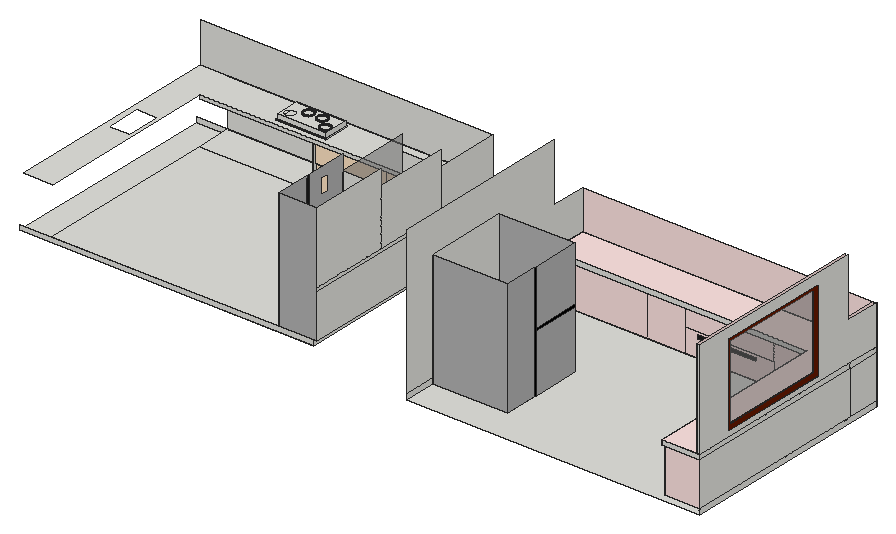
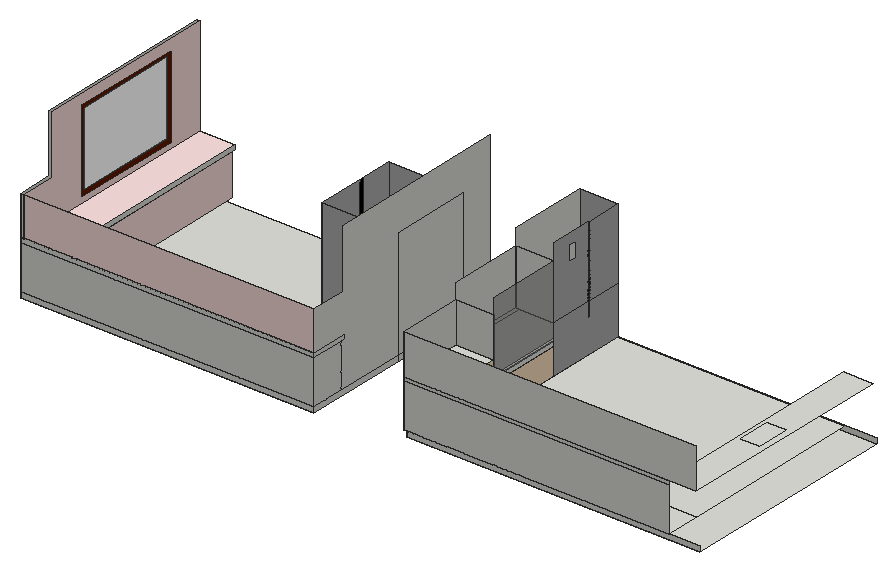
# SketchUp Ruby script. Lengths in inches.
U = 1.inch
M = Sketchup.active_model
def pt(a) = Geom::Point3d.new(a.map { |v| v * U })
def face(e, loops, mat)
  f = e.add_face(loops[0].map { |a| pt(a) })
  loops[1..].each { |l| e.add_face(l.map { |a| pt(a) }).erase! }
  f.material = f.back_material = mat if mat
  f
end
# faces: each face lists its corners as indices into pts; further lists are holes
def faces(e, pts, list, mat = nil) = list.each { |f| face(e, (f[0].is_a?(Array) ? f : [f]).map { |l| l.map { |i| pts[i] } }, mat) }
# xy, xz, yz: faces in a plane at the given z, y or x. An outline is a flat list of corners, or four numbers for a rectangle; further outlines are holes
def ring(l) = l.size == 4 ? [[l[0], l[1]], [l[2], l[1]], [l[2], l[3]], [l[0], l[3]]] : l.each_slice(2).to_a
def flat(e, list, mat, &to3) = list.each { |f| face(e, (f[0].is_a?(Array) ? f : [f]).map { |l| ring(l).map { |u, v| to3.(u, v) } }, mat) }
def xy(e, z, list, mat = nil) = flat(e, list, mat) { |x, y| [x, y, z] }
def xz(e, y, list, mat = nil) = flat(e, list, mat) { |x, z| [x, y, z] }
def yz(e, x, list, mat = nil) = flat(e, list, mat) { |y, z| [x, y, z] }
def lines(e, pts, list) = list.each { |a, b| e.add_line(pt(pts[a]), pt(pts[b])) }
# prism: a flat outline (further loops are holes) pulled along v
def prism(e, loops, v, mat = nil)
  f = face(e, loops, mat); d = Geom::Vector3d.new(v.map { |x| x * U })
  f.pushpull(f.normal.samedirection?(d) ? d.length : -d.length)
end
def box(e, o, s, mat = nil) = prism(e, [[o, [o[0] + s[0], o[1], o[2]], [o[0] + s[0], o[1] + s[1], o[2]], [o[0], o[1] + s[1], o[2]]]], [0, 0, s[2]], mat)
def at(x, y, z, deg = 0) = Geom::Transformation.translation(pt([x, y, z])) * Geom::Transformation.rotation(ORIGIN, Z_AXIS, deg.degrees)
def axes(o, x, y, z) = Geom::Transformation.new([*x, 0, *y, 0, *z, 0, *pt(o).to_a, 1])
def part(name) = M.definitions.add(name)
# library, detail: a bought-in or finely detailed component or shape, given as its bounding box
def library(name, o, s) = part(name).tap { |d| box(d.entities, o, s) }
def detail(e, o, s) = box(e.add_group.entities, o, s)
def put(e, d, t, mat = nil) = e.add_instance(d, t).tap { |i| i.material = mat if mat }
def group(e, t, mat = nil) = e.add_group.tap { |g| g.transformation = t; g.material = mat if mat }.entities
root = M.entities
M.materials.add("[0007_MistyRose]").color = [255, 228, 225]
M.materials.add("[0012_Bisque]").color = [255, 228, 196]
M.materials.add("[0137_Black]").color = [0, 0, 0]
M.materials.add("[Aluminum]").color = [179, 179, 179]
M.materials.add("[Color B08]").color = [102, 25, 0]
M.materials.add("[Color M08]").color = [30, 30, 30]
M.materials.add("[Translucent Glass Gray]").color = [128, 128, 128]
M.materials["[Translucent Glass Gray]"].alpha = 0.5
xy(root,-15,[[317.62,0,317.62,26.55,379.12,26.55,379.12,94.86,317.62,94.86,317.62,180,557.62,180,557.62,0],[317.62,26.55,379.12,94.86]])
xy(root,-11,[[528.62,0,557.62,152.625],[317.62,152.625,557.62,180]])
xy(root,-4,[[0,2.74,240,182.74]])
xy(root,0,[[25.8125,2.74,211,2.74,211,153.74,177.8125,153.74,177.8125,155.18,119.8125,155.18,119.8125,152.62,118.875,152.62,118.875,153.74,25.8125,153.74],[211,2.74,240,153.74],[240,2.74,242.375,153.74],[118.875,152.62,119.8125,153.74],[25.8125,153.74,119.8125,153.74,119.8125,155.18,177.8125,155.18,177.8125,153.74,240,153.74,240,182.74,25.8125,182.74],
  [240,153.74,242.375,182.74]])
xy(root,20.125,[[119.8125,154.62,177.8125,155.18]],"[Color M08]")
xy(root,21.25,[[119.8125,153.74,177.8125,154.62]],"[Color M08]")
xy(root,25,[[528.62,0,528.62,152.625,317.62,152.625,317.62,180,557.62,180,557.62,0],[526.18,0,528.62,152.625],[317.62,148.375,526.18,152.625]])
xy(root,29,[[555.12,0,557.62,152.625],[555.12,152.625,557.62,180]])
xy(root,29,[[526.18,0,555.12,0,555.12,180,317.62,180,317.62,148.375,526.18,148.375]],"[0007_MistyRose]")
xy(root,32.8,[[555.12,28.8125,557.62,121.25]])
xy(root,36,[[119.8125,152.62,177.8125,153.74],[177.8125,152.62,211,153.74]])
xy(root,39,[[[3.25,2.74,26.71,2.74,26.71,152.62,211,152.62,240,153.74,242.375,153.74,242.375,182.74,3.25,182.74],[84.98,157.35,126.29,178.23],[7.17,83.87,24.36,112.5],[5.34,96.75,5.13,96.8,4.95,96.91,4.79,97.05,4.68,97.23,4.62,97.4375,4.62,97.65,4.67,97.85,4.77,98.04,4.91,98.19,5.1,98.31,5.3,98.36,5.51,98.37,5.72,98.32,5.9,98.22,6.06,98.07,6.17,97.89,6.23,97.6875,6.23,97.48,6.18,97.27,6.08,97.08,5.93,96.93,5.75,96.82,5.55,96.76]],[211,129.67,242.375,129.67,242.375,153.74,240,153.74,211,152.62]])
xy(root,39.4375,[[84.98,157.35,126.29,158.42],[85.73,158.42,125.41,178.23],[125.41,158.42,126.29,178.23]])
xy(root,42.875,[[[85.73,158.42,125.41,178.23],[90.7,160.04,89.6,160.26,88.59,160.76,87.74,161.51,87.12,162.44,86.76,163.51,86.6875,164.63,86.91,165.74,87.41,166.75,88.15,167.59,89.09,168.22,90.16,168.58,91.28,168.65,92.38,168.43,93.39,167.93,94.24,167.18,94.86,166.25,95.22,165.18,95.29,164.06,95.07,162.95,94.57,161.94,93.83,161.1,92.89,160.47,91.83,160.11],[100.1,167.5,99,167.73,97.99,168.22,97.14,168.97,96.52,169.9,96.16,170.97,96.09,172.09,96.31,173.2,96.81,174.21,97.55,175.05,98.49,175.68,99.55,176.04,100.68,176.11,101.78,175.89,102.79,175.39,103.64,174.65,104.26,173.71,104.62,172.64,104.69,171.52,104.47,170.42,103.97,169.41,103.23,168.5625,102.29,167.9375,101.22,167.58],[111.41,167.5,110.31,167.73,109.3,168.22,108.46,168.97,107.83,169.9,107.47,170.97,107.4,172.09,107.62,173.2,108.12,174.21,108.86,175.05,109.8,175.68,110.87,176.04,111.99,176.11,113.09,175.89,114.1,175.39,114.95,174.65,115.57,173.71,115.93,172.64,116,171.52,115.78,170.42,115.28,169.41,114.54,168.5625,113.6,167.9375,112.54,167.58],[120.23,159.18,119.13,159.4,118.12,159.9,117.27,160.65,116.65,161.58,116.29,162.65,116.22,163.77,116.4375,164.875,116.9375,165.89,117.68,166.73,118.62,167.35,119.68,167.72,120.81,167.79,121.91,167.57,122.92,167.07,123.77,166.32,124.39,165.39,124.75,164.32,124.82,163.2,124.6,162.09,124.1,161.08,123.36,160.24,122.42,159.61,121.35,159.25]],[120.26,159.61,121.27,159.68,122.23,160,123.07,160.5625,123.74,161.32,124.19,162.23,124.39,163.23,124.33,164.24,124,165.2,123.44,166.04,122.68,166.71,121.77,167.16,120.78,167.36,119.77,167.29,118.81,166.97,117.96,166.41,117.29,165.65,116.85,164.74,116.65,163.74,116.71,162.73,117.04,161.77,117.6,160.93,118.36,160.26,119.27,159.8125],[100.14,168.05,101.12,168.12,102.05,168.43,102.87,168.97,103.52,169.71,103.95,170.59,104.14,171.56,104.08,172.54,103.77,173.47,103.22,174.28,102.48,174.93,101.6,175.37,100.64,175.5625,99.66,175.5,98.73,175.18,97.91,174.64,97.26,173.9,96.83,173.02,96.63,172.06,96.7,171.08,97.01,170.15,97.56,169.33,98.29,168.68,99.17,168.25],[111.46,168.13,112.42,168.19,113.33,168.5,114.13,169.03,114.76,169.76,115.1875,170.62,115.38,171.5625,115.32,172.52,115.01,173.43,114.48,174.23,113.75,174.87,112.89,175.29,111.95,175.48,110.99,175.42,110.08,175.11,109.28,174.58,108.64,173.86,108.21,173,108.02,172.05,108.09,171.09,108.39,170.18,108.93,169.38,109.65,168.75,110.51,168.32]])
xy(root,42.875,[[[120.23,159.18,119.13,159.4,118.12,159.9,117.27,160.65,116.65,161.58,116.29,162.65,116.22,163.77,116.4375,164.875,116.9375,165.89,117.68,166.73,118.62,167.35,119.68,167.72,120.81,167.79,121.91,167.57,122.92,167.07,123.77,166.32,124.39,165.39,124.75,164.32,124.82,163.2,124.6,162.09,124.1,161.08,123.36,160.24,122.42,159.61,121.35,159.25],[120.26,159.61,121.27,159.68,122.23,160,123.07,160.5625,123.74,161.32,124.19,162.23,124.39,163.23,124.33,164.24,124,165.2,123.44,166.04,122.68,166.71,121.77,167.16,120.78,167.36,119.77,167.29,118.81,166.97,117.96,166.41,117.29,165.65,116.85,164.74,116.65,163.74,116.71,162.73,117.04,161.77,117.6,160.93,118.36,160.26,119.27,159.8125]],[[100.1,167.5,99,167.73,97.99,168.22,97.14,168.97,96.52,169.9,96.16,170.97,96.09,172.09,96.31,173.2,96.81,174.21,97.55,175.05,98.49,175.68,99.55,176.04,100.68,176.11,101.78,175.89,102.79,175.39,103.64,174.65,104.26,173.71,104.62,172.64,104.69,171.52,104.47,170.42,103.97,169.41,103.23,168.5625,102.29,167.9375,101.22,167.58],[100.14,168.05,101.12,168.12,102.05,168.43,102.87,168.97,103.52,169.71,103.95,170.59,104.14,171.56,104.08,172.54,103.77,173.47,103.22,174.28,102.48,174.93,101.6,175.37,100.64,175.5625,99.66,175.5,98.73,175.18,97.91,174.64,97.26,173.9,96.83,173.02,96.63,172.06,96.7,171.08,97.01,170.15,97.56,169.33,98.29,168.68,99.17,168.25]],[[111.41,167.5,110.31,167.73,109.3,168.22,108.46,168.97,107.83,169.9,107.47,170.97,107.4,172.09,107.62,173.2,108.12,174.21,108.86,175.05,109.8,175.68,110.87,176.04,111.99,176.11,113.09,175.89,114.1,175.39,114.95,174.65,115.57,173.71,115.93,172.64,116,171.52,115.78,170.42,115.28,169.41,114.54,168.5625,113.6,167.9375,112.54,167.58],[111.46,168.13,112.42,168.19,113.33,168.5,114.13,169.03,114.76,169.76,115.1875,170.62,115.38,171.5625,115.32,172.52,115.01,173.43,114.48,174.23,113.75,174.87,112.89,175.29,111.95,175.48,110.99,175.42,110.08,175.11,109.28,174.58,108.64,173.86,108.21,173,108.02,172.05,108.09,171.09,108.39,170.18,108.93,169.38,109.65,168.75,110.51,168.32]]],"[Color M08]")
xy(root,43.3125,[[[120.23,159.18,121.35,159.25,122.42,159.61,123.36,160.24,124.1,161.08,124.6,162.09,124.82,163.2,124.75,164.32,124.39,165.39,123.77,166.32,122.92,167.07,121.91,167.57,120.81,167.79,119.68,167.72,118.62,167.35,117.68,166.73,116.9375,165.89,116.4375,164.875,116.22,163.77,116.29,162.65,116.65,161.58,117.27,160.65,118.12,159.9,119.13,159.4],[120.26,159.61,119.27,159.8125,118.36,160.26,117.6,160.93,117.04,161.77,116.71,162.73,116.65,163.74,116.85,164.74,117.29,165.65,117.96,166.41,118.81,166.97,119.77,167.29,120.78,167.36,121.77,167.16,122.68,166.71,123.44,166.04,124,165.2,124.33,164.24,124.39,163.23,124.19,162.23,123.74,161.32,123.07,160.5625,122.23,160,121.27,159.68]],[[100.1,167.5,101.22,167.58,102.29,167.9375,103.23,168.5625,103.97,169.41,104.47,170.42,104.69,171.52,104.62,172.64,104.26,173.71,103.64,174.65,102.79,175.39,101.78,175.89,100.68,176.11,99.55,176.04,98.49,175.68,97.55,175.05,96.81,174.21,96.31,173.2,96.09,172.09,96.16,170.97,96.52,169.9,97.14,168.97,97.99,168.22,99,167.73],[100.14,168.05,99.17,168.25,98.29,168.68,97.56,169.33,97.01,170.15,96.7,171.08,96.63,172.06,96.83,173.02,97.26,173.9,97.91,174.64,98.73,175.18,99.66,175.5,100.64,175.5625,101.6,175.37,102.48,174.93,103.22,174.28,103.77,173.47,104.08,172.54,104.14,171.56,103.95,170.59,103.52,169.71,102.87,168.97,102.05,168.43,101.12,168.12]],[[111.41,167.5,112.54,167.58,113.6,167.9375,114.54,168.5625,115.28,169.41,115.78,170.42,116,171.52,115.93,172.64,115.57,173.71,114.95,174.65,114.1,175.39,113.09,175.89,111.99,176.11,110.87,176.04,109.8,175.68,108.86,175.05,108.12,174.21,107.62,173.2,107.4,172.09,107.47,170.97,107.83,169.9,108.46,168.97,109.3,168.22,110.31,167.73],[111.46,168.13,110.51,168.32,109.65,168.75,108.93,169.38,108.39,170.18,108.09,171.09,108.02,172.05,108.21,173,108.64,173.86,109.28,174.58,110.08,175.11,110.99,175.42,111.95,175.48,112.89,175.29,113.75,174.87,114.48,174.23,115.01,173.43,115.32,172.52,115.38,171.5625,115.1875,170.62,114.76,169.76,114.13,169.03,113.33,168.5,112.42,168.19]]],"[Color M08]")
xz(root,0,[[526.18,25,557.62,29],[555.12,29,557.62,109]])
xz(root,0,[[528.62,-11,557.62,25]],"[0007_MistyRose]")
xz(root,2.74,[[0,-4,240,0]])
xz(root,2.74,[[211,0,242.375,97.3125]],"[Aluminum]")
xz(root,26.55,[[317.62,-15,379.12,79.3125]],"[Aluminum]")
xz(root,28.8125,[[555.12,32.8,557.62,100.98]])
xz(root,68.21,[[211,39,242.375,84.66]])
xz(root,94.86,[[317.62,-15,379.12,79.3125]],"[Aluminum]")
xz(root,121.25,[[555.12,32.8,557.62,100.98]])
xz(root,129.67,[[211,39,242.375,72]])
xz(root,148.375,[[317.62,25,526.18,29]])
xz(root,152.62,[[118.875,0,119.8125,36],[26.71,36,211,39]])
xz(root,152.625,[[317.62,-11,392.29,25],[392.29,-11,422.69,25],[[422.69,-11,496.05,8.1],[433.79,3.45,481.16,6.08]],[496.05,-11,528.62,25],[422.69,8.1,496.05,25]],"[0007_MistyRose]")
xz(root,152.625,[[433.79,3.45,481.16,6.08]],"[Color M08]")
xz(root,153.74,[[177.8125,0,211,36],[119.8125,21.25,177.8125,36]],"[0012_Bisque]")
xz(root,154.62,[[119.8125,20.125,177.8125,21.25]],"[Color M08]")
xz(root,155.18,[[119.8125,0,177.8125,20.125]],"[0012_Bisque]")
xz(root,157.35,[[84.98,39,126.29,39.4375]])
xz(root,158.42,[[85.73,39.4375,125.41,42.875]])
xz(root,178.23,[[84.98,39,126.29,39.4375],[85.73,39.4375,125.41,42.875]])
xz(root,180,[[317.62,-15,557.62,-11],[317.62,-11,557.62,25],[317.62,25,557.62,29],[555.12,29,557.62,61]])
xz(root,180,[[317.62,29,555.12,61]],"[0007_MistyRose]")
xz(root,182.74,[[0,-4,240,0],[25.8125,0,242.375,36],[25.8125,36,242.375,39],[3.25,39,242.375,72]])
yz(root,118.875,[[152.62,0,152.62,36,153.74,36,153.74,21.25,154.62,21.25,154.62,20.125,153.74,20.125,153.74,0]])
yz(root,119.8125,[[152.62,0,155.18,0,155.18,20.125,154.62,20.125,154.62,21.25,153.74,21.25,153.74,36,152.62,36]])
yz(root,125.41,[[158.42,39.4375,178.23,42.875]])
yz(root,126.29,[[157.35,39,178.23,39.4375]])
yz(root,177.8125,[[153.74,0,155.18,20.125],[153.74,20.125,154.62,21.25]])
yz(root,211,[[68.21,0,68.21,21.3125,129.67,21.3125,129.67,39,152.62,39,152.62,36,153.74,36,153.74,0]],"[0012_Bisque]")
yz(root,211,[[2.74,0,2.74,39,31.96,39,31.96,27.21,33.15,27.21,33.15,39,68.21,39,68.21,0],[2.74,39,31.96,97.3125],[[33.15,39,68.21,97.3125],[45.79,76.95,53.47,89.39]]],"[Aluminum]")
yz(root,211,[[31.96,27.21,33.15,39],[31.96,39,33.15,97.3125]],"[Color M08]")
yz(root,211,[[68.21,21.3125,129.67,84.66]],"[Translucent Glass Gray]")
yz(root,240,[[2.74,-4,182.74,0]])
yz(root,242.375,[[2.74,0,153.74,36],[153.74,0,182.74,36],[2.74,36,153.74,39],[153.74,36,182.74,39],[2.74,39,68.21,97.3125],
  [68.21,39,129.67,84.66],[129.67,39,182.74,72]])
yz(root,317.62,[[0,-15,26.55,-11],[26.55,-15,94.86,-11],[94.86,-15,180,-11],[0,-11,0,109,151,109,151,61,180,61,180,29,148.375,29,148.375,25,152.625,25,152.625,-11,94.86,-11,94.86,79.3125,26.55,79.3125,26.55,-11],[26.55,-11,94.86,79.3125],
  [152.625,-11,180,25],[148.375,25,180,29]])
yz(root,379.12,[[53.19,-15,55.9,79.3125],[55.9,32.16,94.86,34.55]],"[0137_Black]")
yz(root,379.12,[[26.55,-15,53.19,79.3125],[55.9,-15,94.86,32.16],[55.9,34.55,94.86,79.3125]],"[Aluminum]")
yz(root,526.18,[[0,25,148.375,29]])
yz(root,528.62,[[0,-11,152.625,25]],"[0007_MistyRose]")
yz(root,555.12,[[[0,29,0,109,151,109,151,61,180,61,180,29],[28.8125,32.8,121.25,100.98]]],"[0007_MistyRose]")
yz(root,557.62,[[0,-15,180,-11],[0,-11,152.625,25],[152.625,-11,180,25],[0,25,152.625,29],[152.625,25,180,29],
  [[0,29,180,29,180,61,151,61,151,109,0,109],[28.8125,32.8,121.25,100.98]]])
p = [[119.13,159.4,42.875],[120.23,159.18,42.875],[120.23,159.18,43.3125],[119.13,159.4,43.3125],[121.35,159.25,42.875],[121.35,159.25,43.3125],
  [122.42,159.61,42.875],[122.42,159.61,43.3125],[118.12,159.9,42.875],[118.12,159.9,43.3125],[120.26,159.61,42.875],[119.27,159.8125,42.875],
  [119.27,159.8125,43.3125],[120.26,159.61,43.3125],[121.27,159.68,42.875],[121.27,159.68,43.3125],[123.36,160.24,42.875],[123.36,160.24,43.3125],
  [122.23,160,42.875],[122.23,160,43.3125],[118.36,160.26,42.875],[118.36,160.26,43.3125],[117.27,160.65,42.875],[117.27,160.65,43.3125],
  [123.07,160.5625,42.875],[123.07,160.5625,43.3125],[124.1,161.08,42.875],[124.1,161.08,43.3125],[117.6,160.93,42.875],[117.6,160.93,43.3125],
  [116.65,161.58,42.875],[116.65,161.58,43.3125],[123.74,161.32,42.875],[123.74,161.32,43.3125],[117.04,161.77,42.875],[117.04,161.77,43.3125],
  [124.6,162.09,42.875],[124.6,162.09,43.3125],[124.19,162.23,42.875],[124.19,162.23,43.3125],[116.29,162.65,42.875],[116.29,162.65,43.3125],
  [116.71,162.73,42.875],[116.71,162.73,43.3125],[124.82,163.2,42.875],[124.82,163.2,43.3125],[124.39,163.23,42.875],[124.39,163.23,43.3125],
  [116.22,163.77,42.875],[116.22,163.77,43.3125],[116.65,163.74,42.875],[116.65,163.74,43.3125],[124.33,164.24,42.875],[124.33,164.24,43.3125],
  [124.75,164.32,42.875],[124.75,164.32,43.3125],[116.85,164.74,42.875],[116.85,164.74,43.3125],[116.4375,164.875,42.875],[116.4375,164.875,43.3125],
  [124,165.2,42.875],[124,165.2,43.3125],[124.39,165.39,42.875],[124.39,165.39,43.3125],[117.29,165.65,42.875],[117.29,165.65,43.3125],
  [116.9375,165.89,42.875],[116.9375,165.89,43.3125],[123.44,166.04,42.875],[123.44,166.04,43.3125],[123.77,166.32,42.875],[123.77,166.32,43.3125],
  [117.96,166.41,42.875],[117.96,166.41,43.3125],[117.68,166.73,42.875],[117.68,166.73,43.3125],[122.68,166.71,42.875],[122.68,166.71,43.3125],
  [122.92,167.07,42.875],[122.92,167.07,43.3125],[118.81,166.97,42.875],[118.81,166.97,43.3125],[118.62,167.35,42.875],[118.62,167.35,43.3125],
  [121.77,167.16,42.875],[121.77,167.16,43.3125],[119.77,167.29,42.875],[119.77,167.29,43.3125],[121.91,167.57,42.875],[121.91,167.57,43.3125],
  [120.78,167.36,42.875],[120.78,167.36,43.3125],[119.68,167.72,42.875],[119.68,167.72,43.3125],[99,167.73,42.875],[100.1,167.5,42.875],
  [100.1,167.5,43.3125],[99,167.73,43.3125],[101.22,167.58,42.875],[101.22,167.58,43.3125],[110.31,167.73,42.875],[111.41,167.5,42.875],
  [111.41,167.5,43.3125],[110.31,167.73,43.3125],[112.54,167.58,42.875],[112.54,167.58,43.3125],[102.29,167.9375,42.875],[102.29,167.9375,43.3125],
  [113.6,167.9375,42.875],[113.6,167.9375,43.3125],[120.81,167.79,42.875],[120.81,167.79,43.3125],[97.99,168.22,42.875],[97.99,168.22,43.3125],
  [109.3,168.22,42.875],[109.3,168.22,43.3125],[103.23,168.5625,42.875],[103.23,168.5625,43.3125],[114.54,168.5625,42.875],[114.54,168.5625,43.3125],
  [100.14,168.05,42.875],[99.17,168.25,42.875],[99.17,168.25,43.3125],[100.14,168.05,43.3125],[101.12,168.12,42.875],[101.12,168.12,43.3125],
  [102.05,168.43,42.875],[102.05,168.43,43.3125],[111.46,168.13,42.875],[110.51,168.32,42.875],[110.51,168.32,43.3125],[111.46,168.13,43.3125],
  [112.42,168.19,42.875],[112.42,168.19,43.3125],[97.14,168.97,42.875],[97.14,168.97,43.3125],[98.29,168.68,42.875],[98.29,168.68,43.3125],
  [108.46,168.97,42.875],[108.46,168.97,43.3125],[113.33,168.5,42.875],[113.33,168.5,43.3125],[109.65,168.75,42.875],[109.65,168.75,43.3125],
  [102.87,168.97,42.875],[102.87,168.97,43.3125],[114.13,169.03,42.875],[114.13,169.03,43.3125],[103.97,169.41,42.875],[103.97,169.41,43.3125],
  [115.28,169.41,42.875],[115.28,169.41,43.3125],[97.56,169.33,42.875],[97.56,169.33,43.3125],[108.93,169.38,42.875],[108.93,169.38,43.3125],
  [96.52,169.9,42.875],[96.52,169.9,43.3125],[103.52,169.71,42.875],[103.52,169.71,43.3125],[107.83,169.9,42.875],[107.83,169.9,43.3125],
  [114.76,169.76,42.875],[114.76,169.76,43.3125],[97.01,170.15,42.875],[97.01,170.15,43.3125],[104.47,170.42,42.875],[104.47,170.42,43.3125],
  [108.39,170.18,42.875],[108.39,170.18,43.3125],[115.78,170.42,42.875],[115.78,170.42,43.3125],[103.95,170.59,42.875],[103.95,170.59,43.3125],
  [115.1875,170.62,42.875],[115.1875,170.62,43.3125],[107.47,170.97,42.875],[107.47,170.97,43.3125],[96.7,171.08,42.875],[96.7,171.08,43.3125],
  [108.09,171.09,42.875],[108.09,171.09,43.3125],[104.69,171.52,42.875],[104.69,171.52,43.3125],[116,171.52,42.875],[116,171.52,43.3125],
  [104.14,171.56,42.875],[104.14,171.56,43.3125],[115.38,171.5625,42.875],[115.38,171.5625,43.3125],[107.4,172.09,42.875],[107.4,172.09,43.3125],
  [96.63,172.06,42.875],[96.63,172.06,43.3125],[108.02,172.05,42.875],[108.02,172.05,43.3125],[104.62,172.64,42.875],[104.62,172.64,43.3125],
  [115.93,172.64,42.875],[115.93,172.64,43.3125],[104.08,172.54,42.875],[104.08,172.54,43.3125],[115.32,172.52,42.875],[115.32,172.52,43.3125],
  [96.83,173.02,42.875],[96.83,173.02,43.3125],[107.62,173.2,42.875],[107.62,173.2,43.3125],[108.21,173,42.875],[108.21,173,43.3125],
  [103.77,173.47,42.875],[103.77,173.47,43.3125],[115.01,173.43,42.875],[115.01,173.43,43.3125],[104.26,173.71,42.875],[104.26,173.71,43.3125],
  [115.57,173.71,42.875],[115.57,173.71,43.3125],[97.26,173.9,42.875],[97.26,173.9,43.3125],[108.64,173.86,42.875],[108.64,173.86,43.3125],
  [108.12,174.21,42.875],[108.12,174.21,43.3125],[114.48,174.23,42.875],[114.48,174.23,43.3125],[103.22,174.28,42.875],[103.22,174.28,43.3125],
  [103.64,174.65,42.875],[103.64,174.65,43.3125],[114.95,174.65,42.875],[114.95,174.65,43.3125],[97.91,174.64,42.875],[97.91,174.64,43.3125],
  [109.28,174.58,42.875],[109.28,174.58,43.3125],[97.55,175.05,42.875],[96.81,174.21,42.875],[96.81,174.21,43.3125],[97.55,175.05,43.3125],
  [108.86,175.05,42.875],[108.86,175.05,43.3125],[113.75,174.87,42.875],[113.75,174.87,43.3125],[102.48,174.93,42.875],[102.48,174.93,43.3125],
  [98.73,175.18,42.875],[98.73,175.18,43.3125],[102.79,175.39,42.875],[102.79,175.39,43.3125],[110.08,175.11,42.875],[110.08,175.11,43.3125],
  [114.1,175.39,42.875],[114.1,175.39,43.3125],[101.6,175.37,42.875],[101.6,175.37,43.3125],[112.89,175.29,42.875],[112.89,175.29,43.3125],
  [98.49,175.68,42.875],[98.49,175.68,43.3125],[109.8,175.68,42.875],[109.8,175.68,43.3125],[110.99,175.42,42.875],[110.99,175.42,43.3125],
  [99.66,175.5,42.875],[99.66,175.5,43.3125],[111.95,175.48,42.875],[111.95,175.48,43.3125],[100.64,175.5625,42.875],[100.64,175.5625,43.3125],
  [101.78,175.89,42.875],[101.78,175.89,43.3125],[113.09,175.89,42.875],[113.09,175.89,43.3125],[99.55,176.04,42.875],[99.55,176.04,43.3125],
  [110.87,176.04,42.875],[110.87,176.04,43.3125],[100.68,176.11,42.875],[100.68,176.11,43.3125],[111.99,176.11,42.875],[111.99,176.11,43.3125],
  [557.62,0,-11],[557.62,-1.5,-11]]
faces(root,p,[[0,1,2,3],[1,4,5,2],[4,6,7,5],[8,0,3,9],[10,11,12,13],[14,10,13,15],[6,16,17,7],[18,14,15,19],
  [11,20,21,12],[22,8,9,23],[24,18,19,25],[16,26,27,17],[20,28,29,21],[30,22,23,31],[32,24,25,33],[28,34,35,29],
  [26,36,37,27],[38,32,33,39],[40,30,31,41],[34,42,43,35],[36,44,45,37],[46,38,39,47],[48,40,41,49],[42,50,51,43],
  [52,46,47,53],[44,54,55,45],[50,56,57,51],[58,48,49,59],[60,52,53,61],[54,62,63,55],[56,64,65,57],[66,58,59,67],
  [68,60,61,69],[62,70,71,63],[64,72,73,65],[74,66,67,75],[76,68,69,77],[70,78,79,71],[72,80,81,73],[82,74,75,83],
  [84,76,77,85],[80,86,87,81],[78,88,89,79],[90,84,85,91],[86,90,91,87],[92,82,83,93],[94,95,96,97],[95,98,99,96],
  [100,101,102,103],[101,104,105,102],[98,106,107,99],[104,108,109,105],[88,110,111,89],[112,94,97,113],[114,100,103,115],[110,92,93,111],
  [106,116,117,107],[108,118,119,109],[120,121,122,123],[124,120,123,125],[126,124,125,127],[128,129,130,131],[132,128,131,133],[134,112,113,135],
  [121,136,137,122],[138,114,115,139],[140,132,133,141],[129,142,143,130],[144,126,127,145],[146,140,141,147],[116,148,149,117],[118,150,151,119],
  [136,152,153,137],[142,154,155,143],[156,134,135,157],[158,144,145,159],[160,138,139,161],[162,146,147,163],[152,164,165,153],[148,166,167,149],
  [154,168,169,155],[150,170,171,151],[172,158,159,173],[174,162,163,175],[176,160,161,177],[164,178,179,165],[168,180,181,169],[166,182,183,167],
  [170,184,185,171],[186,172,173,187],[188,174,175,189],[190,176,177,191],[178,192,193,179],[180,194,195,181],[182,196,197,183],[184,198,199,185],
  [200,186,187,201],[202,188,189,203],[192,204,205,193],[206,190,191,207],[194,208,209,195],[210,200,201,211],[212,202,203,213],[196,214,215,197],
  [198,216,217,199],[204,218,219,205],[208,220,221,209],[222,206,207,223],[224,212,213,225],[226,210,211,227],[214,228,229,215],[216,230,231,217],
  [218,232,233,219],[220,234,235,221],[236,237,238,239],[240,222,223,241],[242,224,225,243],[244,226,227,245],[232,246,247,233],[228,248,249,229],
  [234,250,251,235],[230,252,253,231],[254,244,245,255],[256,242,243,257],[258,236,239,259],[260,240,241,261],[250,262,263,251],[246,264,265,247],
  [266,256,257,267],[268,254,255,269],[248,270,271,249],[262,266,267,263],[252,272,273,253],[264,268,269,265],[274,258,259,275],[276,260,261,277],
  [270,278,279,271],[272,280,281,273],[278,274,275,279],[280,276,277,281]],"[Color M08]")
lines(root,p,[[282,283]])
g1 = group(root,at(556.46,28.8125,32.8))
xy(g1,0,[[-1.28,0,0,92.4375]],"[Color B08]")
xy(g1,3.53,[[-1.28,3.26,0,89.18]],"[Color B08]")
xy(g1,64.66,[[-1.28,3.26,0,89.18]],"[Color B08]")
xy(g1,68.1875,[[-1.28,0,0,92.4375]],"[Color B08]")
xz(g1,0,[[-1.28,0,0,68.1875]],"[Color B08]")
xz(g1,3.26,[[-1.28,3.53,0,64.66]],"[Color B08]")
xz(g1,89.18,[[-1.28,3.53,0,64.66]],"[Color B08]")
xz(g1,92.4375,[[-1.28,0,0,68.1875]],"[Color B08]")
yz(g1,-1.28,[[[0,0,92.4375,68.1875],[3.26,3.53,89.18,64.66]]],"[Color B08]")
yz(g1,-1.28,[[3.26,3.53,89.18,64.66]],"[Translucent Glass Gray]")
yz(g1,0,[[[0,0,92.4375,68.1875],[3.26,3.53,89.18,64.66]]],"[Color B08]")
